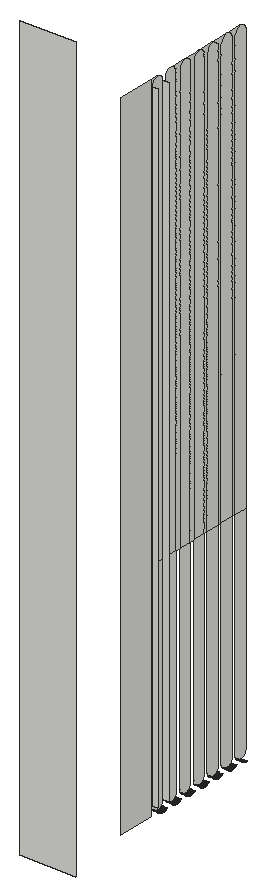
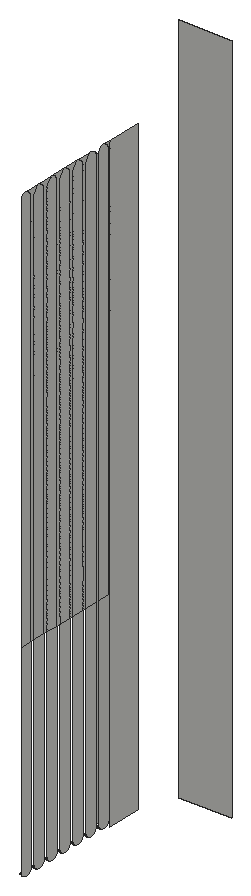
# SketchUp Ruby script. Lengths in inches.
U = 1.inch
M = Sketchup.active_model
def pt(a) = Geom::Point3d.new(a.map { |v| v * U })
def face(e, loops, mat)
  f = e.add_face(loops[0].map { |a| pt(a) })
  loops[1..].each { |l| e.add_face(l.map { |a| pt(a) }).erase! }
  f.material = f.back_material = mat if mat
  f
end
# faces: each face lists its corners as indices into pts; further lists are holes
def faces(e, pts, list, mat = nil) = list.each { |f| face(e, (f[0].is_a?(Array) ? f : [f]).map { |l| l.map { |i| pts[i] } }, mat) }
# xy, xz, yz: faces in a plane at the given z, y or x. An outline is a flat list of corners, or four numbers for a rectangle; further outlines are holes
def ring(l) = l.size == 4 ? [[l[0], l[1]], [l[2], l[1]], [l[2], l[3]], [l[0], l[3]]] : l.each_slice(2).to_a
def flat(e, list, mat, &to3) = list.each { |f| face(e, (f[0].is_a?(Array) ? f : [f]).map { |l| ring(l).map { |u, v| to3.(u, v) } }, mat) }
def xy(e, z, list, mat = nil) = flat(e, list, mat) { |x, y| [x, y, z] }
def xz(e, y, list, mat = nil) = flat(e, list, mat) { |x, z| [x, y, z] }
def yz(e, x, list, mat = nil) = flat(e, list, mat) { |y, z| [x, y, z] }
def lines(e, pts, list) = list.each { |a, b| e.add_line(pt(pts[a]), pt(pts[b])) }
# prism: a flat outline (further loops are holes) pulled along v
def prism(e, loops, v, mat = nil)
  f = face(e, loops, mat); d = Geom::Vector3d.new(v.map { |x| x * U })
  f.pushpull(f.normal.samedirection?(d) ? d.length : -d.length)
end
def box(e, o, s, mat = nil) = prism(e, [[o, [o[0] + s[0], o[1], o[2]], [o[0] + s[0], o[1] + s[1], o[2]], [o[0], o[1] + s[1], o[2]]]], [0, 0, s[2]], mat)
def at(x, y, z, deg = 0) = Geom::Transformation.translation(pt([x, y, z])) * Geom::Transformation.rotation(ORIGIN, Z_AXIS, deg.degrees)
def axes(o, x, y, z) = Geom::Transformation.new([*x, 0, *y, 0, *z, 0, *pt(o).to_a, 1])
def part(name) = M.definitions.add(name)
# library, detail: a bought-in or finely detailed component or shape, given as its bounding box
def library(name, o, s) = part(name).tap { |d| box(d.entities, o, s) }
def detail(e, o, s) = box(e.add_group.entities, o, s)
def put(e, d, t, mat = nil) = e.add_instance(d, t).tap { |i| i.material = mat if mat }
def group(e, t, mat = nil) = e.add_group.tap { |g| g.transformation = t; g.material = mat if mat }.entities
root = M.entities
xz(root,0,[[0,0,9,120]])
xz(root,15.231,[[9,3.521,10,106.961]])
xz(root,17.3125,[[9,3.521,10,106.961]])
yz(root,9,[[9,2,15,108],[16.272,2.396,16.329,2.398,16.386,2.403,16.443,2.41,16.499,2.421,16.555,2.435,16.61,2.452,16.663,2.473,16.716,2.495,16.767,2.521,16.817,2.55,16.865,2.581,16.911,2.615,16.956,2.651,16.998,2.69,17.038,2.731,17.076,2.774,17.111,2.82,17.144,2.867,17.174,2.915,17.202,2.966,17.226,3.018,17.248,3.071,17.267,3.125,17.283,3.18,17.295,3.236,17.305,3.292,17.3125,3.363,17.3125,38,15.231,38,15.231,3.363,15.238,3.292,15.248,3.236,15.261,3.18,15.277,3.125,15.295,3.071,15.317,3.018,15.342,2.966,15.369,2.915,15.4,2.867,15.432,2.82,15.468,2.774,15.505,2.731,15.546,2.69,15.588,2.651,15.632,2.615,15.678,2.581,15.727,2.55,15.776,2.521,15.827,2.495,15.88,2.473,15.934,2.452,15.989,2.435,16.044,2.421,16.1,2.41,16.157,2.403,16.214,2.398],[19.059,2.396,19.117,2.398,19.174,2.403,19.231,2.41,19.287,2.421,19.342,2.435,19.397,2.452,19.451,2.473,19.504,2.495,19.555,2.521,19.604,2.55,19.653,2.581,19.699,2.615,19.743,2.651,19.785,2.69,19.826,2.731,19.863,2.774,19.899,2.82,19.931,2.867,19.962,2.915,19.989,2.966,20.014,3.018,20.036,3.071,20.054,3.125,20.07,3.18,20.083,3.236,20.093,3.292,20.1,3.363,20.1,38,18.018,38,18.018,3.363,18.026,3.292,18.036,3.236,18.048,3.18,18.064,3.125,18.083,3.071,18.105,3.018,18.129,2.966,18.157,2.915,18.187,2.867,18.22,2.82,18.255,2.774,18.293,2.731,18.333,2.69,18.375,2.651,18.42,2.615,18.466,2.581,18.514,2.55,18.564,2.521,18.615,2.495,18.668,2.473,18.721,2.452,18.776,2.435,18.832,2.421,18.888,2.41,18.945,2.403,19.002,2.398],[21.847,2.396,21.904,2.398,21.961,2.403,22.018,2.41,22.074,2.421,22.13,2.435,22.185,2.452,22.238,2.473,22.291,2.495,22.342,2.521,22.392,2.55,22.44,2.581,22.486,2.615,22.531,2.651,22.573,2.69,22.613,2.731,22.651,2.774,22.686,2.82,22.719,2.867,22.749,2.915,22.777,2.966,22.801,3.018,22.823,3.071,22.842,3.125,22.858,3.18,22.87,3.236,22.88,3.292,22.887,3.363,22.887,38,20.806,38,20.806,3.363,20.813,3.292,20.823,3.236,20.836,3.18,20.852,3.125,20.87,3.071,20.892,3.018,20.917,2.966,20.944,2.915,20.975,2.867,21.007,2.82,21.043,2.774,21.08,2.731,21.121,2.69,21.163,2.651,21.207,2.615,21.253,2.581,21.302,2.55,21.351,2.521,21.402,2.495,21.455,2.473,21.509,2.452,21.564,2.435,21.619,2.421,21.675,2.41,21.732,2.403,21.789,2.398],[24.634,2.396,24.692,2.398,24.749,2.403,24.806,2.41,24.862,2.421,24.917,2.435,24.972,2.452,25.026,2.473,25.079,2.495,25.13,2.521,25.179,2.55,25.228,2.581,25.274,2.615,25.318,2.651,25.36,2.69,25.401,2.731,25.438,2.774,25.474,2.82,25.506,2.867,25.537,2.915,25.564,2.966,25.589,3.018,25.611,3.071,25.629,3.125,25.645,3.18,25.658,3.236,25.668,3.292,25.675,3.363,25.675,38,23.593,38,23.593,3.363,23.601,3.292,23.611,3.236,23.623,3.18,23.639,3.125,23.658,3.071,23.68,3.018,23.704,2.966,23.732,2.915,23.762,2.867,23.795,2.82,23.83,2.774,23.868,2.731,23.908,2.69,23.95,2.651,23.995,2.615,24.041,2.581,24.089,2.55,24.139,2.521,24.19,2.495,24.243,2.473,24.296,2.452,24.351,2.435,24.407,2.421,24.463,2.41,24.52,2.403,24.577,2.398],
  [27.422,2.396,27.479,2.398,27.536,2.403,27.593,2.41,27.649,2.421,27.705,2.435,27.76,2.452,27.813,2.473,27.866,2.495,27.917,2.521,27.967,2.55,28.015,2.581,28.061,2.615,28.106,2.651,28.148,2.69,28.188,2.731,28.226,2.774,28.261,2.82,28.294,2.867,28.324,2.915,28.352,2.966,28.376,3.018,28.398,3.071,28.417,3.125,28.433,3.18,28.445,3.236,28.455,3.292,28.462,3.363,28.462,38,26.381,38,26.381,3.363,26.388,3.292,26.398,3.236,26.411,3.18,26.427,3.125,26.445,3.071,26.467,3.018,26.492,2.966,26.519,2.915,26.55,2.867,26.582,2.82,26.618,2.774,26.655,2.731,26.696,2.69,26.738,2.651,26.782,2.615,26.828,2.581,26.877,2.55,26.926,2.521,26.977,2.495,27.03,2.473,27.084,2.452,27.139,2.435,27.194,2.421,27.25,2.41,27.307,2.403,27.364,2.398],[30.209,2.396,30.267,2.398,30.324,2.403,30.381,2.41,30.437,2.421,30.492,2.435,30.547,2.452,30.601,2.473,30.654,2.495,30.705,2.521,30.754,2.55,30.803,2.581,30.849,2.615,30.893,2.651,30.935,2.69,30.976,2.731,31.013,2.774,31.049,2.82,31.081,2.867,31.112,2.915,31.139,2.966,31.164,3.018,31.186,3.071,31.204,3.125,31.22,3.18,31.233,3.236,31.243,3.292,31.25,3.363,31.25,38,29.168,38,29.168,3.363,29.176,3.292,29.186,3.236,29.198,3.18,29.214,3.125,29.233,3.071,29.255,3.018,29.279,2.966,29.307,2.915,29.337,2.867,29.37,2.82,29.405,2.774,29.443,2.731,29.483,2.69,29.525,2.651,29.57,2.615,29.616,2.581,29.664,2.55,29.714,2.521,29.765,2.495,29.818,2.473,29.871,2.452,29.926,2.435,29.982,2.421,30.038,2.41,30.095,2.403,30.152,2.398],[32.997,2.396,33.054,2.398,33.111,2.403,33.168,2.41,33.224,2.421,33.28,2.435,33.335,2.452,33.388,2.473,33.441,2.495,33.492,2.521,33.542,2.55,33.59,2.581,33.636,2.615,33.681,2.651,33.723,2.69,33.763,2.731,33.801,2.774,33.836,2.82,33.869,2.867,33.899,2.915,33.927,2.966,33.951,3.018,33.973,3.071,33.992,3.125,34.008,3.18,34.02,3.236,34.03,3.292,34.037,3.363,34.037,38,31.956,38,31.956,3.363,31.963,3.292,31.973,3.236,31.986,3.18,32.002,3.125,32.02,3.071,32.042,3.018,32.067,2.966,32.094,2.915,32.125,2.867,32.157,2.82,32.193,2.774,32.23,2.731,32.271,2.69,32.313,2.651,32.357,2.615,32.403,2.581,32.452,2.55,32.501,2.521,32.552,2.495,32.605,2.473,32.659,2.452,32.714,2.435,32.769,2.421,32.825,2.41,32.882,2.403,32.939,2.398],[15.231,3.363,15.231,3.521,15.228,3.464,15.228,3.407],[17.3125,3.363,17.315,3.407,17.315,3.464,17.3125,3.521],
  [18.018,3.363,18.018,3.521,18.016,3.464,18.016,3.407],[20.1,3.363,20.103,3.407,20.103,3.464,20.1,3.521],[20.806,3.363,20.806,3.521,20.803,3.464,20.803,3.407],[22.887,3.363,22.89,3.407,22.89,3.464,22.887,3.521],[23.593,3.363,23.593,3.521,23.591,3.464,23.591,3.407],
  [25.675,3.363,25.678,3.407,25.678,3.464,25.675,3.521],[26.381,3.363,26.381,3.521,26.378,3.464,26.378,3.407],[28.462,3.363,28.465,3.407,28.465,3.464,28.462,3.521],[29.168,3.363,29.168,3.521,29.166,3.464,29.166,3.407],[31.25,3.363,31.253,3.407,31.253,3.464,31.25,3.521],
  [31.956,3.363,31.956,3.521,31.953,3.464,31.953,3.407],[15,38,15.231,38,15.231,106.961,15.232,107.015,15.237,107.069,15.244,107.123,15.254,107.177,15.266,107.23,15.282,107.282,15.3,107.334,15.321,107.384,15.344,107.433,15.37,107.481,15.399,107.528,15.43,107.572,15.463,107.616,15.498,107.657,15.536,107.697,15.575,107.734,15.617,107.769,15.66,107.803,15.705,107.834,15.751,107.862,15.799,107.888,15.848,107.911,15.899,107.932,15.95,107.95,16.002,107.966,16.055,107.979,16.109,107.989,16.163,107.996,16.217,108,15,108],[15.231,38,17.3125,38,17.3125,106.961,17.311,107.015,17.307,107.069,17.3,107.123,17.29,107.177,17.277,107.23,17.262,107.282,17.243,107.334,17.223,107.384,17.199,107.433,17.173,107.481,17.145,107.528,17.114,107.572,17.081,107.616,17.045,107.657,17.008,107.697,16.968,107.734,16.927,107.769,16.883,107.803,16.839,107.834,16.792,107.862,16.744,107.888,16.695,107.911,16.645,107.932,16.593,107.95,16.541,107.966,16.488,107.979,16.435,107.989,16.381,107.996,16.326,108,16.217,108,16.163,107.996,16.109,107.989,16.055,107.979,16.002,107.966,15.95,107.95,15.899,107.932,15.848,107.911,15.799,107.888,15.751,107.862,15.705,107.834,15.66,107.803,15.617,107.769,15.575,107.734,15.536,107.697,15.498,107.657,15.463,107.616,15.43,107.572,15.399,107.528,15.37,107.481,15.344,107.433,15.321,107.384,15.3,107.334,15.282,107.282,15.266,107.23,15.254,107.177,15.244,107.123,15.237,107.069,15.232,107.015,15.231,106.961],[18.018,38,20.1,38,20.1,106.961,20.099,107.015,20.094,107.069,20.087,107.123,20.077,107.177,20.065,107.23,20.049,107.282,20.031,107.334,20.01,107.384,19.987,107.433,19.961,107.481,19.932,107.528,19.901,107.572,19.868,107.616,19.833,107.657,19.795,107.697,19.756,107.734,19.714,107.769,19.671,107.803,19.626,107.834,19.58,107.862,19.532,107.888,19.483,107.911,19.432,107.932,19.381,107.95,19.329,107.966,19.276,107.979,19.222,107.989,19.168,107.996,19.114,108,19.005,108,18.95,107.996,18.896,107.989,18.843,107.979,18.79,107.966,18.738,107.95,18.686,107.932,18.636,107.911,18.587,107.888,18.539,107.862,18.492,107.834,18.448,107.803,18.404,107.769,18.363,107.734,18.323,107.697,18.286,107.657,18.25,107.616,18.217,107.572,18.186,107.528,18.158,107.481,18.132,107.433,18.108,107.384,18.088,107.334,18.069,107.282,18.054,107.23,18.041,107.177,18.031,107.123,18.024,107.069,18.02,107.015,18.018,106.961],[20.1,38,20.806,38,20.806,106.961,20.807,107.015,20.812,107.069,20.819,107.123,20.829,107.177,20.841,107.23,20.857,107.282,20.875,107.334,20.896,107.384,20.919,107.433,20.945,107.481,20.974,107.528,21.005,107.572,21.038,107.616,21.073,107.657,21.111,107.697,21.15,107.734,21.192,107.769,21.235,107.803,21.28,107.834,21.326,107.862,21.374,107.888,21.423,107.911,21.474,107.932,21.525,107.95,21.577,107.966,21.63,107.979,21.684,107.989,21.738,107.996,21.792,108,19.114,108,19.168,107.996,19.222,107.989,19.276,107.979,19.329,107.966,19.381,107.95,19.432,107.932,19.483,107.911,19.532,107.888,19.58,107.862,19.626,107.834,19.671,107.803,19.714,107.769,19.756,107.734,19.795,107.697,19.833,107.657,19.868,107.616,19.901,107.572,19.932,107.528,19.961,107.481,19.987,107.433,20.01,107.384,20.031,107.334,20.049,107.282,20.065,107.23,20.077,107.177,20.087,107.123,20.094,107.069,20.099,107.015,20.1,106.961],
  [20.806,38,22.887,38,22.887,106.961,22.886,107.015,22.882,107.069,22.875,107.123,22.865,107.177,22.852,107.23,22.837,107.282,22.818,107.334,22.798,107.384,22.774,107.433,22.748,107.481,22.72,107.528,22.689,107.572,22.656,107.616,22.62,107.657,22.583,107.697,22.543,107.734,22.502,107.769,22.458,107.803,22.414,107.834,22.367,107.862,22.319,107.888,22.27,107.911,22.22,107.932,22.168,107.95,22.116,107.966,22.063,107.979,22.01,107.989,21.956,107.996,21.901,108,21.792,108,21.738,107.996,21.684,107.989,21.63,107.979,21.577,107.966,21.525,107.95,21.474,107.932,21.423,107.911,21.374,107.888,21.326,107.862,21.28,107.834,21.235,107.803,21.192,107.769,21.15,107.734,21.111,107.697,21.073,107.657,21.038,107.616,21.005,107.572,20.974,107.528,20.945,107.481,20.919,107.433,20.896,107.384,20.875,107.334,20.857,107.282,20.841,107.23,20.829,107.177,20.819,107.123,20.812,107.069,20.807,107.015,20.806,106.961],[22.887,38,23.593,38,23.593,106.961,23.595,107.015,23.599,107.069,23.606,107.123,23.616,107.177,23.629,107.23,23.644,107.282,23.663,107.334,23.683,107.384,23.707,107.433,23.733,107.481,23.761,107.528,23.792,107.572,23.825,107.616,23.861,107.657,23.898,107.697,23.938,107.734,23.979,107.769,24.023,107.803,24.067,107.834,24.114,107.862,24.162,107.888,24.211,107.911,24.261,107.932,24.3125,107.95,24.365,107.966,24.418,107.979,24.471,107.989,24.525,107.996,24.58,108,21.901,108,21.956,107.996,22.01,107.989,22.063,107.979,22.116,107.966,22.168,107.95,22.22,107.932,22.27,107.911,22.319,107.888,22.367,107.862,22.414,107.834,22.458,107.803,22.502,107.769,22.543,107.734,22.583,107.697,22.62,107.657,22.656,107.616,22.689,107.572,22.72,107.528,22.748,107.481,22.774,107.433,22.798,107.384,22.818,107.334,22.837,107.282,22.852,107.23,22.865,107.177,22.875,107.123,22.882,107.069,22.886,107.015,22.887,106.961],[23.593,38,25.675,38,25.675,106.961,25.674,107.015,25.669,107.069,25.662,107.123,25.652,107.177,25.64,107.23,25.624,107.282,25.606,107.334,25.585,107.384,25.562,107.433,25.536,107.481,25.507,107.528,25.476,107.572,25.443,107.616,25.408,107.657,25.37,107.697,25.331,107.734,25.289,107.769,25.246,107.803,25.201,107.834,25.155,107.862,25.107,107.888,25.058,107.911,25.007,107.932,24.956,107.95,24.904,107.966,24.851,107.979,24.797,107.989,24.743,107.996,24.689,108,24.58,108,24.525,107.996,24.471,107.989,24.418,107.979,24.365,107.966,24.3125,107.95,24.261,107.932,24.211,107.911,24.162,107.888,24.114,107.862,24.067,107.834,24.023,107.803,23.979,107.769,23.938,107.734,23.898,107.697,23.861,107.657,23.825,107.616,23.792,107.572,23.761,107.528,23.733,107.481,23.707,107.433,23.683,107.384,23.663,107.334,23.644,107.282,23.629,107.23,23.616,107.177,23.606,107.123,23.599,107.069,23.595,107.015,23.593,106.961],[25.675,38,26.381,38,26.381,106.961,26.382,107.015,26.387,107.069,26.394,107.123,26.404,107.177,26.416,107.23,26.432,107.282,26.45,107.334,26.471,107.384,26.494,107.433,26.52,107.481,26.549,107.528,26.58,107.572,26.613,107.616,26.648,107.657,26.686,107.697,26.725,107.734,26.767,107.769,26.81,107.803,26.855,107.834,26.901,107.862,26.949,107.888,26.998,107.911,27.049,107.932,27.1,107.95,27.152,107.966,27.205,107.979,27.259,107.989,27.313,107.996,27.367,108,24.689,108,24.743,107.996,24.797,107.989,24.851,107.979,24.904,107.966,24.956,107.95,25.007,107.932,25.058,107.911,25.107,107.888,25.155,107.862,25.201,107.834,25.246,107.803,25.289,107.769,25.331,107.734,25.37,107.697,25.408,107.657,25.443,107.616,25.476,107.572,25.507,107.528,25.536,107.481,25.562,107.433,25.585,107.384,25.606,107.334,25.624,107.282,25.64,107.23,25.652,107.177,25.662,107.123,25.669,107.069,25.674,107.015,25.675,106.961],[26.381,38,28.462,38,28.462,106.961,28.461,107.015,28.457,107.069,28.45,107.123,28.44,107.177,28.427,107.23,28.412,107.282,28.393,107.334,28.373,107.384,28.349,107.433,28.323,107.481,28.295,107.528,28.264,107.572,28.231,107.616,28.195,107.657,28.158,107.697,28.118,107.734,28.077,107.769,28.033,107.803,27.989,107.834,27.942,107.862,27.894,107.888,27.845,107.911,27.795,107.932,27.743,107.95,27.691,107.966,27.638,107.979,27.585,107.989,27.531,107.996,27.476,108,27.367,108,27.313,107.996,27.259,107.989,27.205,107.979,27.152,107.966,27.1,107.95,27.049,107.932,26.998,107.911,26.949,107.888,26.901,107.862,26.855,107.834,26.81,107.803,26.767,107.769,26.725,107.734,26.686,107.697,26.648,107.657,26.613,107.616,26.58,107.572,26.549,107.528,26.52,107.481,26.494,107.433,26.471,107.384,26.45,107.334,26.432,107.282,26.416,107.23,26.404,107.177,26.394,107.123,26.387,107.069,26.382,107.015,26.381,106.961],
  [28.462,38,29.168,38,29.168,106.961,29.17,107.015,29.174,107.069,29.181,107.123,29.191,107.177,29.204,107.23,29.219,107.282,29.238,107.334,29.258,107.384,29.282,107.433,29.308,107.481,29.336,107.528,29.367,107.572,29.4,107.616,29.436,107.657,29.473,107.697,29.513,107.734,29.554,107.769,29.598,107.803,29.642,107.834,29.689,107.862,29.737,107.888,29.786,107.911,29.836,107.932,29.888,107.95,29.94,107.966,29.993,107.979,30.046,107.989,30.1,107.996,30.155,108,27.476,108,27.531,107.996,27.585,107.989,27.638,107.979,27.691,107.966,27.743,107.95,27.795,107.932,27.845,107.911,27.894,107.888,27.942,107.862,27.989,107.834,28.033,107.803,28.077,107.769,28.118,107.734,28.158,107.697,28.195,107.657,28.231,107.616,28.264,107.572,28.295,107.528,28.323,107.481,28.349,107.433,28.373,107.384,28.393,107.334,28.412,107.282,28.427,107.23,28.44,107.177,28.45,107.123,28.457,107.069,28.461,107.015,28.462,106.961],[29.168,38,31.25,38,31.25,106.961,31.249,107.015,31.244,107.069,31.237,107.123,31.227,107.177,31.215,107.23,31.199,107.282,31.181,107.334,31.16,107.384,31.137,107.433,31.111,107.481,31.082,107.528,31.051,107.572,31.018,107.616,30.983,107.657,30.945,107.697,30.906,107.734,30.864,107.769,30.821,107.803,30.776,107.834,30.73,107.862,30.682,107.888,30.633,107.911,30.582,107.932,30.531,107.95,30.479,107.966,30.426,107.979,30.372,107.989,30.318,107.996,30.264,108,30.155,108,30.1,107.996,30.046,107.989,29.993,107.979,29.94,107.966,29.888,107.95,29.836,107.932,29.786,107.911,29.737,107.888,29.689,107.862,29.642,107.834,29.598,107.803,29.554,107.769,29.513,107.734,29.473,107.697,29.436,107.657,29.4,107.616,29.367,107.572,29.336,107.528,29.308,107.481,29.282,107.433,29.258,107.384,29.238,107.334,29.219,107.282,29.204,107.23,29.191,107.177,29.181,107.123,29.174,107.069,29.17,107.015,29.168,106.961],[31.25,38,31.956,38,31.956,106.961,31.957,107.015,31.962,107.069,31.969,107.123,31.979,107.177,31.991,107.23,32.007,107.282,32.025,107.334,32.046,107.384,32.069,107.433,32.095,107.481,32.124,107.528,32.155,107.572,32.188,107.616,32.223,107.657,32.261,107.697,32.3,107.734,32.342,107.769,32.385,107.803,32.43,107.834,32.476,107.862,32.524,107.888,32.573,107.911,32.624,107.932,32.675,107.95,32.727,107.966,32.78,107.979,32.834,107.989,32.888,107.996,32.942,108,30.264,108,30.318,107.996,30.372,107.989,30.426,107.979,30.479,107.966,30.531,107.95,30.582,107.932,30.633,107.911,30.682,107.888,30.73,107.862,30.776,107.834,30.821,107.803,30.864,107.769,30.906,107.734,30.945,107.697,30.983,107.657,31.018,107.616,31.051,107.572,31.082,107.528,31.111,107.481,31.137,107.433,31.16,107.384,31.181,107.334,31.199,107.282,31.215,107.23,31.227,107.177,31.237,107.123,31.244,107.069,31.249,107.015,31.25,106.961],[31.956,38,34.037,38,34.037,106.961,34.036,107.015,34.032,107.069,34.025,107.123,34.015,107.177,34.002,107.23,33.987,107.282,33.968,107.334,33.948,107.384,33.924,107.433,33.898,107.481,33.87,107.528,33.839,107.572,33.806,107.616,33.77,107.657,33.733,107.697,33.693,107.734,33.652,107.769,33.608,107.803,33.564,107.834,33.517,107.862,33.469,107.888,33.42,107.911,33.37,107.932,33.318,107.95,33.266,107.966,33.213,107.979,33.16,107.989,33.106,107.996,33.051,108,32.942,108,32.888,107.996,32.834,107.989,32.78,107.979,32.727,107.966,32.675,107.95,32.624,107.932,32.573,107.911,32.524,107.888,32.476,107.862,32.43,107.834,32.385,107.803,32.342,107.769,32.3,107.734,32.261,107.697,32.223,107.657,32.188,107.616,32.155,107.572,32.124,107.528,32.095,107.481,32.069,107.433,32.046,107.384,32.025,107.334,32.007,107.282,31.991,107.23,31.979,107.177,31.969,107.123,31.962,107.069,31.957,107.015,31.956,106.961]])
p = [[9,15.934,2.452],[9,15.989,2.435],[10,15.989,2.435],[10,15.934,2.452],[9,16.044,2.421],[10,16.044,2.421],
  [9,16.1,2.41],[10,16.1,2.41],[9,16.157,2.403],[10,16.157,2.403],[9,16.214,2.398],[10,16.214,2.398],
  [9,16.272,2.396],[10,16.272,2.396],[9,16.329,2.398],[10,16.329,2.398],[9,16.386,2.403],[10,16.386,2.403],
  [9,16.443,2.41],[10,16.443,2.41],[9,16.499,2.421],[10,16.499,2.421],[9,16.555,2.435],[10,16.555,2.435],
  [9,16.61,2.452],[10,16.61,2.452],[9,18.721,2.452],[9,18.776,2.435],[10,18.776,2.435],[10,18.721,2.452],
  [9,18.832,2.421],[10,18.832,2.421],[9,18.888,2.41],[10,18.888,2.41],[9,18.945,2.403],[10,18.945,2.403],
  [9,19.002,2.398],[10,19.002,2.398],[9,19.059,2.396],[10,19.059,2.396],[9,19.117,2.398],[10,19.117,2.398],
  [9,19.174,2.403],[10,19.174,2.403],[9,19.231,2.41],[10,19.231,2.41],[9,19.287,2.421],[10,19.287,2.421],
  [9,19.342,2.435],[10,19.342,2.435],[9,19.397,2.452],[10,19.397,2.452],[9,21.509,2.452],[9,21.564,2.435],
  [10,21.564,2.435],[10,21.509,2.452],[9,21.619,2.421],[10,21.619,2.421],[9,21.675,2.41],[10,21.675,2.41],
  [9,21.732,2.403],[10,21.732,2.403],[9,21.789,2.398],[10,21.789,2.398],[9,21.847,2.396],[10,21.847,2.396],
  [9,21.904,2.398],[10,21.904,2.398],[9,21.961,2.403],[10,21.961,2.403],[9,22.018,2.41],[10,22.018,2.41],
  [9,22.074,2.421],[10,22.074,2.421],[9,22.13,2.435],[10,22.13,2.435],[9,22.185,2.452],[10,22.185,2.452],
  [9,24.296,2.452],[9,24.351,2.435],[10,24.351,2.435],[10,24.296,2.452],[9,24.407,2.421],[10,24.407,2.421],
  [9,24.463,2.41],[10,24.463,2.41],[9,24.52,2.403],[10,24.52,2.403],[9,24.577,2.398],[10,24.577,2.398],
  [9,24.634,2.396],[10,24.634,2.396],[9,24.692,2.398],[10,24.692,2.398],[9,24.749,2.403],[10,24.749,2.403],
  [9,24.806,2.41],[10,24.806,2.41],[9,24.862,2.421],[10,24.862,2.421],[9,24.917,2.435],[10,24.917,2.435],
  [9,24.972,2.452],[10,24.972,2.452],[9,27.084,2.452],[9,27.139,2.435],[10,27.139,2.435],[10,27.084,2.452],
  [9,27.194,2.421],[10,27.194,2.421],[9,27.25,2.41],[10,27.25,2.41],[9,27.307,2.403],[10,27.307,2.403],
  [9,27.364,2.398],[10,27.364,2.398],[9,27.422,2.396],[10,27.422,2.396],[9,27.479,2.398],[10,27.479,2.398],
  [9,27.536,2.403],[10,27.536,2.403],[9,27.593,2.41],[10,27.593,2.41],[9,27.649,2.421],[10,27.649,2.421],
  [9,27.705,2.435],[10,27.705,2.435],[9,27.76,2.452],[10,27.76,2.452],[9,29.871,2.452],[9,29.926,2.435],
  [10,29.926,2.435],[10,29.871,2.452],[9,29.982,2.421],[10,29.982,2.421],[9,30.038,2.41],[10,30.038,2.41],
  [9,30.095,2.403],[10,30.095,2.403],[9,30.152,2.398],[10,30.152,2.398],[9,30.209,2.396],[10,30.209,2.396],
  [9,30.267,2.398],[10,30.267,2.398],[9,30.324,2.403],[10,30.324,2.403],[9,30.381,2.41],[10,30.381,2.41],
  [9,30.437,2.421],[10,30.437,2.421],[9,30.492,2.435],[10,30.492,2.435],[9,30.547,2.452],[10,30.547,2.452],
  [9,32.659,2.452],[9,32.714,2.435],[10,32.714,2.435],[10,32.659,2.452],[9,32.769,2.421],[10,32.769,2.421],
  [9,32.825,2.41],[10,32.825,2.41],[9,32.882,2.403],[10,32.882,2.403],[9,32.939,2.398],[10,32.939,2.398],
  [9,32.997,2.396],[10,32.997,2.396],[9,33.054,2.398],[10,33.054,2.398],[9,15.678,2.581],[9,15.727,2.55],
  [10,15.727,2.55],[10,15.678,2.581],[9,15.776,2.521],[10,15.776,2.521],[9,15.827,2.495],[10,15.827,2.495],
  [9,15.88,2.473],[10,15.88,2.473],[9,16.663,2.473],[10,16.663,2.473],[9,16.716,2.495],[10,16.716,2.495],
  [9,16.767,2.521],[10,16.767,2.521],[9,16.817,2.55],[10,16.817,2.55],[9,16.865,2.581],[10,16.865,2.581],
  [9,18.466,2.581],[9,18.514,2.55],[10,18.514,2.55],[10,18.466,2.581],[9,18.564,2.521],[10,18.564,2.521],
  [9,18.615,2.495],[10,18.615,2.495],[9,18.668,2.473],[10,18.668,2.473],[9,19.451,2.473],[10,19.451,2.473],
  [9,19.504,2.495],[10,19.504,2.495],[9,19.555,2.521],[10,19.555,2.521],[9,19.604,2.55],[10,19.604,2.55],
  [9,19.653,2.581],[10,19.653,2.581],[9,21.253,2.581],[9,21.302,2.55],[10,21.302,2.55],[10,21.253,2.581],
  [9,21.351,2.521],[10,21.351,2.521],[9,21.402,2.495],[10,21.402,2.495],[9,21.455,2.473],[10,21.455,2.473],
  [9,22.238,2.473],[10,22.238,2.473],[9,22.291,2.495],[10,22.291,2.495],[9,22.342,2.521],[10,22.342,2.521],
  [9,22.392,2.55],[10,22.392,2.55],[9,22.44,2.581],[10,22.44,2.581],[9,24.041,2.581],[9,24.089,2.55],
  [10,24.089,2.55],[10,24.041,2.581],[9,24.139,2.521],[10,24.139,2.521],[9,24.19,2.495],[10,24.19,2.495],
  [9,24.243,2.473],[10,24.243,2.473],[9,25.026,2.473],[10,25.026,2.473],[9,25.079,2.495],[10,25.079,2.495],
  [9,25.13,2.521],[10,25.13,2.521],[9,25.179,2.55],[10,25.179,2.55],[9,25.228,2.581],[10,25.228,2.581],
  [9,26.828,2.581],[9,26.877,2.55],[10,26.877,2.55],[10,26.828,2.581],[9,26.926,2.521],[10,26.926,2.521],
  [9,26.977,2.495],[10,26.977,2.495],[9,27.03,2.473],[10,27.03,2.473],[9,27.813,2.473],[10,27.813,2.473],
  [9,27.866,2.495],[10,27.866,2.495],[9,27.917,2.521],[10,27.917,2.521],[9,27.967,2.55],[10,27.967,2.55],
  [9,28.015,2.581],[10,28.015,2.581],[9,29.616,2.581],[9,29.664,2.55],[10,29.664,2.55],[10,29.616,2.581],
  [9,29.714,2.521],[10,29.714,2.521],[9,29.765,2.495],[10,29.765,2.495],[9,29.818,2.473],[10,29.818,2.473],
  [9,30.601,2.473],[10,30.601,2.473],[9,30.654,2.495],[10,30.654,2.495],[9,30.705,2.521],[10,30.705,2.521],
  [9,30.754,2.55],[10,30.754,2.55],[9,30.803,2.581],[10,30.803,2.581],[9,32.403,2.581],[9,32.452,2.55],
  [10,32.452,2.55],[10,32.403,2.581],[9,32.501,2.521],[10,32.501,2.521],[9,32.552,2.495],[10,32.552,2.495],
  [9,32.605,2.473],[10,32.605,2.473],[9,15.588,2.651],[9,15.632,2.615],[10,15.632,2.615],[10,15.588,2.651],
  [9,16.911,2.615],[10,16.911,2.615],[9,16.956,2.651],[10,16.956,2.651],[9,18.375,2.651],[9,18.42,2.615],
  [10,18.42,2.615],[10,18.375,2.651],[9,19.699,2.615],[10,19.699,2.615],[9,19.743,2.651],[10,19.743,2.651],
  [9,21.163,2.651],[9,21.207,2.615],[10,21.207,2.615],[10,21.163,2.651],[9,22.486,2.615],[10,22.486,2.615],
  [9,22.531,2.651],[10,22.531,2.651],[9,23.95,2.651],[9,23.995,2.615],[10,23.995,2.615],[10,23.95,2.651],
  [9,25.274,2.615],[10,25.274,2.615],[9,25.318,2.651],[10,25.318,2.651],[9,26.738,2.651],[9,26.782,2.615],
  [10,26.782,2.615],[10,26.738,2.651],[9,28.061,2.615],[10,28.061,2.615],[9,28.106,2.651],[10,28.106,2.651],
  [9,29.525,2.651],[9,29.57,2.615],[10,29.57,2.615],[10,29.525,2.651],[9,30.849,2.615],[10,30.849,2.615],
  [9,30.893,2.651],[10,30.893,2.651],[9,32.313,2.651],[9,32.357,2.615],[10,32.357,2.615],[10,32.313,2.651],
  [9,15.546,2.69],[10,15.546,2.69],[9,16.998,2.69],[10,16.998,2.69],[9,17.038,2.731],[10,17.038,2.731],
  [9,18.333,2.69],[10,18.333,2.69],[9,19.785,2.69],[10,19.785,2.69],[9,19.826,2.731],[10,19.826,2.731],
  [9,21.121,2.69],[10,21.121,2.69],[9,22.573,2.69],[10,22.573,2.69],[9,22.613,2.731],[10,22.613,2.731],
  [9,23.908,2.69],[10,23.908,2.69],[9,25.36,2.69],[10,25.36,2.69],[9,25.401,2.731],[10,25.401,2.731],
  [9,26.696,2.69],[10,26.696,2.69],[9,28.148,2.69],[10,28.148,2.69],[9,28.188,2.731],[10,28.188,2.731],
  [9,29.483,2.69],[10,29.483,2.69],[9,30.935,2.69],[10,30.935,2.69],[9,30.976,2.731],[10,30.976,2.731],
  [9,32.271,2.69],[10,32.271,2.69]]
faces(root,p,[[0,1,2,3],[1,4,5,2],[4,6,7,5],[6,8,9,7],[8,10,11,9],[10,12,13,11],[12,14,15,13],[14,16,17,15],
  [16,18,19,17],[18,20,21,19],[20,22,23,21],[22,24,25,23],[26,27,28,29],[27,30,31,28],[30,32,33,31],[32,34,35,33],
  [34,36,37,35],[36,38,39,37],[38,40,41,39],[40,42,43,41],[42,44,45,43],[44,46,47,45],[46,48,49,47],[48,50,51,49],
  [52,53,54,55],[53,56,57,54],[56,58,59,57],[58,60,61,59],[60,62,63,61],[62,64,65,63],[64,66,67,65],[66,68,69,67],
  [68,70,71,69],[70,72,73,71],[72,74,75,73],[74,76,77,75],[78,79,80,81],[79,82,83,80],[82,84,85,83],[84,86,87,85],
  [86,88,89,87],[88,90,91,89],[90,92,93,91],[92,94,95,93],[94,96,97,95],[96,98,99,97],[98,100,101,99],[100,102,103,101],
  [104,105,106,107],[105,108,109,106],[108,110,111,109],[110,112,113,111],[112,114,115,113],[114,116,117,115],[116,118,119,117],[118,120,121,119],
  [120,122,123,121],[122,124,125,123],[124,126,127,125],[126,128,129,127],[130,131,132,133],[131,134,135,132],[134,136,137,135],[136,138,139,137],
  [138,140,141,139],[140,142,143,141],[142,144,145,143],[144,146,147,145],[146,148,149,147],[148,150,151,149],[150,152,153,151],[152,154,155,153],
  [156,157,158,159],[157,160,161,158],[160,162,163,161],[162,164,165,163],[164,166,167,165],[166,168,169,167],[168,170,171,169],[172,173,174,175],
  [173,176,177,174],[176,178,179,177],[178,180,181,179],[180,0,3,181],[24,182,183,25],[182,184,185,183],[184,186,187,185],[186,188,189,187],
  [188,190,191,189],[192,193,194,195],[193,196,197,194],[196,198,199,197],[198,200,201,199],[200,26,29,201],[50,202,203,51],[202,204,205,203],
  [204,206,207,205],[206,208,209,207],[208,210,211,209],[212,213,214,215],[213,216,217,214],[216,218,219,217],[218,220,221,219],[220,52,55,221],
  [76,222,223,77],[222,224,225,223],[224,226,227,225],[226,228,229,227],[228,230,231,229],[232,233,234,235],[233,236,237,234],[236,238,239,237],
  [238,240,241,239],[240,78,81,241],[102,242,243,103],[242,244,245,243],[244,246,247,245],[246,248,249,247],[248,250,251,249],[252,253,254,255],
  [253,256,257,254],[256,258,259,257],[258,260,261,259],[260,104,107,261],[128,262,263,129],[262,264,265,263],[264,266,267,265],[266,268,269,267],
  [268,270,271,269],[272,273,274,275],[273,276,277,274],[276,278,279,277],[278,280,281,279],[280,130,133,281],[154,282,283,155],[282,284,285,283],
  [284,286,287,285],[286,288,289,287],[288,290,291,289],[292,293,294,295],[293,296,297,294],[296,298,299,297],[298,300,301,299],[300,156,159,301],
  [302,303,304,305],[303,172,175,304],[190,306,307,191],[306,308,309,307],[310,311,312,313],[311,192,195,312],[210,314,315,211],[314,316,317,315],
  [318,319,320,321],[319,212,215,320],[230,322,323,231],[322,324,325,323],[326,327,328,329],[327,232,235,328],[250,330,331,251],[330,332,333,331],
  [334,335,336,337],[335,252,255,336],[270,338,339,271],[338,340,341,339],[342,343,344,345],[343,272,275,344],[290,346,347,291],[346,348,349,347],
  [350,351,352,353],[351,292,295,352],[354,302,305,355],[308,356,357,309],[356,358,359,357],[360,310,313,361],[316,362,363,317],[362,364,365,363],
  [366,318,321,367],[324,368,369,325],[368,370,371,369],[372,326,329,373],[332,374,375,333],[374,376,377,375],[378,334,337,379],[340,380,381,341],
  [380,382,383,381],[384,342,345,385],[348,386,387,349],[386,388,389,387],[390,350,353,391]])
